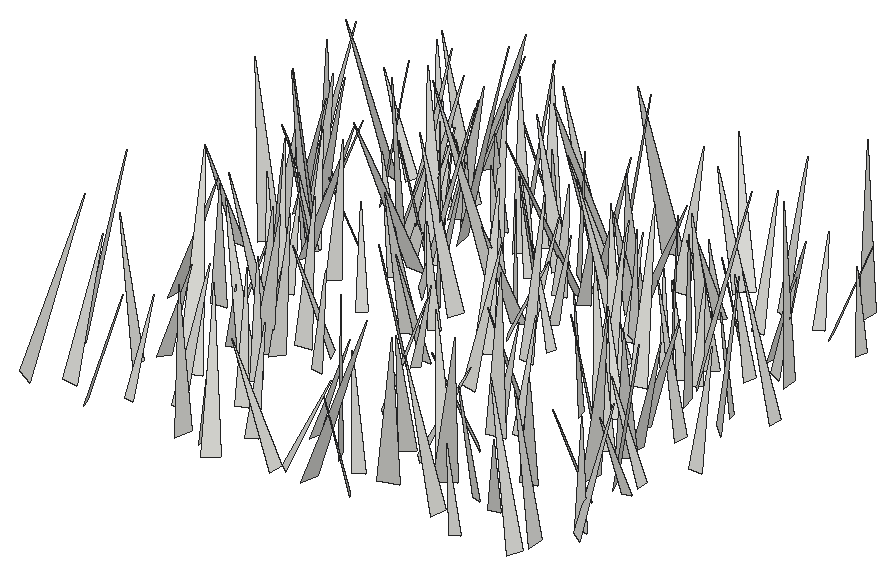
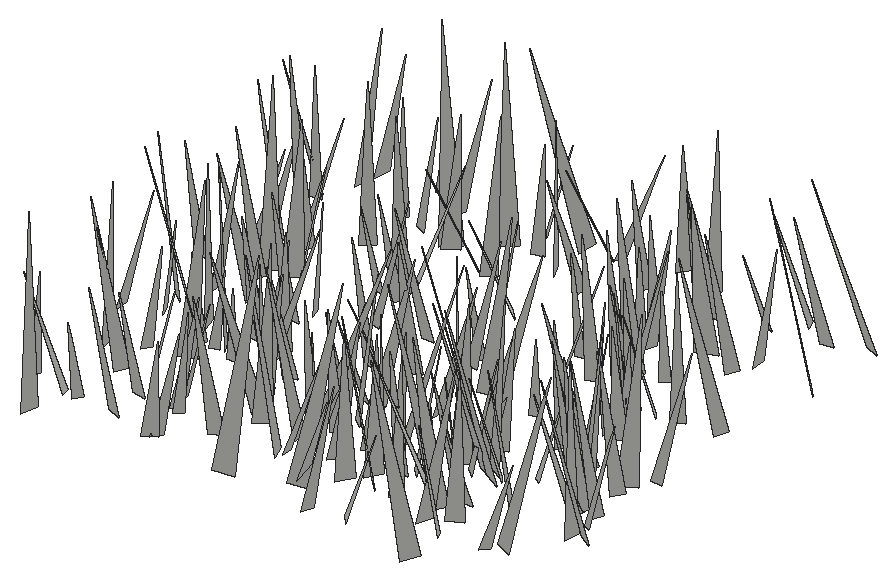
# SketchUp Ruby script. Lengths in inches.
U = 1.inch
M = Sketchup.active_model
def pt(a) = Geom::Point3d.new(a.map { |v| v * U })
def face(e, loops, mat)
  f = e.add_face(loops[0].map { |a| pt(a) })
  loops[1..].each { |l| e.add_face(l.map { |a| pt(a) }).erase! }
  f.material = f.back_material = mat if mat
  f
end
# faces: each face lists its corners as indices into pts; further lists are holes
def faces(e, pts, list, mat = nil) = list.each { |f| face(e, (f[0].is_a?(Array) ? f : [f]).map { |l| l.map { |i| pts[i] } }, mat) }
# xy, xz, yz: faces in a plane at the given z, y or x. An outline is a flat list of corners, or four numbers for a rectangle; further outlines are holes
def ring(l) = l.size == 4 ? [[l[0], l[1]], [l[2], l[1]], [l[2], l[3]], [l[0], l[3]]] : l.each_slice(2).to_a
def flat(e, list, mat, &to3) = list.each { |f| face(e, (f[0].is_a?(Array) ? f : [f]).map { |l| ring(l).map { |u, v| to3.(u, v) } }, mat) }
def xy(e, z, list, mat = nil) = flat(e, list, mat) { |x, y| [x, y, z] }
def xz(e, y, list, mat = nil) = flat(e, list, mat) { |x, z| [x, y, z] }
def yz(e, x, list, mat = nil) = flat(e, list, mat) { |y, z| [x, y, z] }
def lines(e, pts, list) = list.each { |a, b| e.add_line(pt(pts[a]), pt(pts[b])) }
# prism: a flat outline (further loops are holes) pulled along v
def prism(e, loops, v, mat = nil)
  f = face(e, loops, mat); d = Geom::Vector3d.new(v.map { |x| x * U })
  f.pushpull(f.normal.samedirection?(d) ? d.length : -d.length)
end
def box(e, o, s, mat = nil) = prism(e, [[o, [o[0] + s[0], o[1], o[2]], [o[0] + s[0], o[1] + s[1], o[2]], [o[0], o[1] + s[1], o[2]]]], [0, 0, s[2]], mat)
def at(x, y, z, deg = 0) = Geom::Transformation.translation(pt([x, y, z])) * Geom::Transformation.rotation(ORIGIN, Z_AXIS, deg.degrees)
def axes(o, x, y, z) = Geom::Transformation.new([*x, 0, *y, 0, *z, 0, *pt(o).to_a, 1])
def part(name) = M.definitions.add(name)
# library, detail: a bought-in or finely detailed component or shape, given as its bounding box
def library(name, o, s) = part(name).tap { |d| box(d.entities, o, s) }
def detail(e, o, s) = box(e.add_group.entities, o, s)
def put(e, d, t, mat = nil) = e.add_instance(d, t).tap { |i| i.material = mat if mat }
def group(e, t, mat = nil) = e.add_group.tap { |g| g.transformation = t; g.material = mat if mat }.entities
root = M.entities
c1 = part("fur_instance\#9")
p = [[0.8125,0,1.79],[0.67,-0.02,1.48],[0,-0.11,0],[0,0.11,0]]
faces(c1.entities,p,[[0,1,2,3]])
put(root,c1,axes([517.21,158.68,-21.66],[5.69628,-2.00129,2.37758],[-1.98509,-6.1627,-0.4314],[-2.39112,0.34864,6.02217]))
put(root,c1,axes([525.48,158.79,-21.66],[-5.10669,0.68056,0.36828],[0.71376,5.09217,0.48729],[0.29888,-0.53268,5.12875]))
put(root,c1,axes([509.02,157.88,-21.66],[4.30125,1.72732,0.68489],[1.69718,-4.35514,0.32517],[-0.75649,0.05042,4.6237]))
put(root,c1,axes([520.79,157.32,-21.66],[-4.49131,4.50007,0.95246],[4.50728,4.57122,-0.34355],[0.91773,-0.42777,6.34858]))
put(root,c1,axes([531.84,159.24,-21.66],[-3.00946,-2.45302,0.73779],[-2.54129,3.00205,-0.38468],[0.32167,0.76736,3.86344]))
put(root,c1,axes([518.95,158.54,-21.66],[-3.597,-0.64897,1.74683],[-0.97146,3.89365,-0.55385],[1.59023,0.91068,3.61287]))
put(root,c1,axes([541.32,159.27,-21.66],[1.53479,-3.08573,1.52348],[-3.30012,-1.79268,-0.30636],[-0.97569,1.2095,3.43271]))
put(root,c1,axes([528.25,159.17,-21.66],[7.76844,-0.71206,0.72464],[-0.74639,-7.79129,0.34557],[-0.68922,0.41169,7.79335]))
put(root,c1,axes([503.29,158.16,-21.66],[3.5873,6.66463,1.07182],[6.75002,-3.55215,-0.50434],[-0.05834,-1.18311,7.55193]))
put(root,c1,axes([525.89,159.3,-21.66],[2.47782,3.1575,0.0552],[3.13992,-2.45577,-0.47176],[0.33732,-0.3344,3.98583]))
put(root,c1,axes([532.87,162.28,-21.66],[3.4393,-6.56896,1.063],[-6.65437,-3.3911,0.57422],[0.02233,1.20797,7.39258]))
put(root,c1,axes([506.24,159.51,-21.66],[-0.03084,5.75903,1.17934],[5.85206,0.14189,-0.53988],[0.55736,-1.17118,5.73375]))
put(root,c1,axes([538.45,161.01,-21.66],[-6.00997,1.04438,1.22572],[1.13938,6.10462,0.38513],[1.13796,-0.59647,6.08787]))
put(root,c1,axes([546.26,159.875,-21.66],[-6.22467,1.67352,0.58559],[1.62437,6.23957,-0.56507],[0.71064,0.39649,6.42089]))
put(root,c1,axes([546.57,161.78,-21.66],[5.59524,-0.57904,3.08549],[-0.36766,-6.38318,-0.53118],[-3.11775,-0.28642,5.59999]))
put(root,c1,axes([511.12,160.11,-21.66],[1.03899,3.82207,0.22987],[3.79032,-1.06041,0.49963],[-0.54276,-0.08876,3.92914]))
put(root,c1,axes([521.38,161.21,-21.66],[2.89571,-2.97183,2.13904],[-3.49598,-3.05481,0.48854],[-1.08874,1.90494,4.12046]))
put(root,c1,axes([530.41,162.06,-21.66],[1.59272,-3.9303,2.28796],[-4.37909,-1.9795,-0.352],[-1.22702,1.96293,4.22612]))
put(root,c1,axes([541.33,163.7,-21.66],[1.84889,-3.8875,0.07331],[-3.87281,-1.83403,0.41727],[0.34554,0.24513,4.2845]))
put(root,c1,axes([514.63,161.35,-21.66],[0.44242,5.64748,1.29703],[5.78226,-0.34572,-0.46699],[0.37666,-1.32609,5.6455]))
put(root,c1,axes([536,164.81,-21.66],[5.23004,-6.31048,0.45418],[-6.32662,-5.22094,0.31214],[-0.04891,0.54893,8.19012]))
put(root,c1,axes([527.96,163.07,-21.66],[5.01686,3.02729,2.73746],[3.17963,-5.61852,0.38618],[-2.55892,-1.04628,5.84673]))
put(root,c1,axes([539.24,164.29,-21.66],[1.51862,3.68557,2.40948],[4.21899,-1.94756,0.31991],[-1.2606,-2.07817,3.97332]))
put(root,c1,axes([524.69,164.1875,-21.66],[4.46137,-0.22154,0.62784],[-0.29219,-4.4737,0.49769],[-0.59824,0.53291,4.43905]))
put(root,c1,axes([547.81,165.39,-21.66],[0.13174,-4.85064,1.64659],[-5.10405,0.01535,0.4536],[0.43432,1.65178,4.83118]))
put(root,c1,axes([531.17,166.6,-21.66],[3.50702,-4.68842,0.88051],[-4.69288,-3.58696,-0.4079],[-0.85643,0.45629,5.84073]))
put(root,c1,axes([508.36,164.66,-21.66],[-5.56537,0.35389,1.01892],[0.25962,5.63719,-0.53984],[1.04691,0.48332,5.55042]))
put(root,c1,axes([548.24,164.44,-21.66],[2.85218,4.71528,1.10181],[4.83661,-2.83604,-0.38317],[-0.23454,-1.14272,5.49745]))
put(root,c1,axes([517.9375,164.33,-21.66],[-0.91047,5.0165,1.03079],[5.11456,0.83694,0.44447],[-0.2628,-1.09133,5.07905]))
put(root,c1,axes([535.75,165.17,-21.66],[2.97491,-4.25566,3.74848],[-5.0806,-3.88069,-0.37363],[-2.51977,2.80026,5.17891]))
put(root,c1,axes([509.08,166.65,-21.66],[4.36325,-2.68491,0.18726],[-2.69098,-4.34538,0.39756],[0.04948,0.43666,5.1077]))
put(root,c1,axes([502.97,165.3,-21.66],[5.7382,5.20942,1.87337],[5.41352,-5.84467,-0.3291],[-1.15821,-1.50876,7.74318]))
put(root,c1,axes([540.72,168.36,-21.66],[2.46673,-5.38252,0.46134],[-5.39282,-2.42347,0.55987],[0.31917,0.65147,5.89431]))
put(root,c1,axes([532.47,166.27,-21.66],[3.00056,3.161,0.00616],[3.13284,-2.97269,-0.58633],[0.42105,-0.40809,4.31874]))
put(root,c1,axes([545.46,169.32,-21.66],[-2.21382,-3.77344,0.32599],[-3.76288,2.23425,0.30817],[0.43109,0.1241,4.36404]))
put(root,c1,axes([512.21,165.71,-21.66],[-3.14428,7.71271,0.49149],[7.72648,3.12546,0.38342],[-0.17032,-0.59964,8.32018]))
put(root,c1,axes([516.44,167.86,-21.66],[-4.17339,1.81444,1.20525],[1.74242,4.34394,-0.50613],[1.30721,0.0026,4.52253]))
put(root,c1,axes([534.71,170.26,-21.66],[-3.28468,-3.33783,0.1825],[-3.30088,3.27904,0.56182],[0.52783,-0.26523,4.64915]))
put(root,c1,axes([515.92,167.7,-21.66],[-6.2227,2.39174,0.32304],[2.36421,6.22042,-0.51348],[0.48507,0.36431,6.64671]))
put(root,c1,axes([512,170.68,-21.66],[1.97582,-3.11414,0.08334],[-3.10691,-1.9626,0.3224],[0.22782,0.24287,3.67393]))
put(root,c1,axes([547.16,171.4,-21.66],[0.58704,-3.79537,0.45103],[-3.78334,-0.64184,-0.47675],[-0.5428,0.36891,3.81079]))
put(root,c1,axes([514.3125,171.22,-21.66],[4.31409,-4.88001,1.43702],[-5.06352,-4.30068,0.59646],[-0.49016,1.47666,6.48614]))
put(root,c1,axes([543.75,171.66,-21.66],[6.97924,-1.80721,1.76653],[-1.77915,-7.19853,-0.33521],[-1.79479,0.10824,7.20163]))
put(root,c1,axes([526.32,169.87,-21.66],[3.1839,3.43631,0.24845],[3.39454,-3.18669,0.57383],[-0.5891,0.20968,4.64932]))
put(root,c1,axes([518.89,171.69,-21.66],[0.06663,3.86387,1.64805],[4.18879,0.06273,-0.31643],[0.31563,-1.6482,3.85147]))
put(root,c1,axes([545.68,171.99,-21.66],[5.68987,2.39384,1.65752],[2.61602,-5.80047,-0.60296],[-1.2784,-1.21517,6.14342]))
put(root,c1,axes([515.33,171.69,-21.66],[-4.36102,2.95909,2.58691],[3.11538,4.95832,-0.41976],[2.39639,-1.06094,5.25343]))
put(root,c1,axes([534.66,172.28,-21.66],[-1.49682,6.02983,3.22428],[6.74332,1.8484,-0.32627],[1.1325,-3.03643,6.20426]))
put(root,c1,axes([513.74,172.29,-21.66],[3.88682,0.49651,1.01606],[0.42112,-4.01087,0.34905],[-1.04955,0.22945,3.90283]))
put(root,c1,axes([547.17,173.17,-21.66],[-4.29082,0.07848,0.62907],[0.12494,4.3243,0.31276],[0.62151,-0.32753,4.28013]))
put(root,c1,axes([504.15,174.11,-21.66],[6.51578,-0.90085,0.09034],[-0.89347,-6.50413,-0.41604],[-0.1463,-0.39981,6.56459]))
put(root,c1,axes([518.3,174.24,-21.66],[-4.34148,-1.68145,0.56308],[-1.64517,4.37512,0.38015],[0.66161,-0.1544,4.64018]))
put(root,c1,axes([543.86,175.57,-21.66],[3.44417,-6.15496,0.43731],[-6.17002,-3.42915,0.33004],[0.07525,0.54268,7.04535]))
put(root,c1,axes([512.47,174.1875,-21.66],[-6.25427,-0.78477,1.30734],[-0.71032,6.38344,0.43371],[1.34924,-0.27711,6.28838]))
put(root,c1,axes([533.98,173.38,-21.66],[3.92282,-1.4058,1.44453],[-1.66907,-4.03753,0.60333],[-1.1301,1.0833,4.1232]))
put(root,c1,axes([507.6,174.75,-21.66],[1.5026,-5.2869,1.47769],[-5.48951,-1.44343,0.41772],[0.01326,1.53554,5.48039]))
put(root,c1,axes([515.98,173.75,-21.66],[-1.18817,5.57554,2.26119],[5.96275,1.39894,-0.31626],[0.80332,-2.13721,5.69196]))
put(root,c1,axes([535.79,173.29,-21.66],[0.78964,4.34465,0.57519],[4.335,-0.86018,0.54605],[-0.64386,-0.46311,4.38193]))
put(root,c1,axes([511.11,175.375,-21.66],[3.01124,-3.84874,1.35887],[-4.04465,-3.04041,0.35153],[-0.54781,1.29229,4.87409]))
put(root,c1,axes([523.21,176.34,-21.66],[-3.17607,-4.40082,1.193],[-4.40846,3.33508,0.56622],[1.16445,0.62283,5.3976]))
put(root,c1,axes([509.4,174.93,-21.66],[3.16954,2.48643,0.53995],[2.54162,-3.13416,-0.48689],[-0.1185,-0.71733,3.99891]))
put(root,c1,axes([540.9375,175.87,-21.66],[-4.28874,-2.62611,1.19653],[-2.76089,4.3576,-0.33198],[0.84,0.91449,5.01792]))
put(root,c1,axes([532.98,177.26,-21.66],[-1.82356,-4.42835,0.39133],[-4.41286,1.85435,0.42054],[0.53859,0.19978,4.77062]))
put(root,c1,axes([541.95,175.36,-21.66],[-4.3858,5.26104,2.02142],[5.54364,4.48874,0.34523],[1.01623,-1.78118,6.84066]))
put(root,c1,axes([543.71,176.92,-21.66],[5.53978,-0.90724,0.62547],[-0.85463,-5.56113,-0.49688],[-0.69563,-0.39269,5.59154]))
put(root,c1,axes([524.07,177.5,-21.66],[-0.19346,-4.85951,0.89963],[-4.92735,0.1202,-0.41034],[-0.38132,0.91231,4.84602]))
put(root,c1,axes([524.06,176.43,-21.66],[3.08181,-1.73974,0.98019],[-1.88437,-3.1302,0.36886],[-0.66077,0.81254,3.51969]))
put(root,c1,axes([528.84,176.48,-21.66],[0.94432,5.62245,1.27282],[5.76049,-0.87093,-0.42662],[0.22085,-1.32412,5.68522]))
put(root,c1,axes([548.88,177.07,-21.66],[-0.27729,4.76979,1.49646],[4.98187,0.38774,-0.31274],[0.41383,-1.47171,4.7676]))
put(root,c1,axes([510.15,177.32,-21.66],[3.4021,4.35261,1.87369],[4.47593,-3.70904,0.48912],[-1.55627,-1.15238,5.50275]))
put(root,c1,axes([520.65,179.97,-21.66],[2.01145,-6.31603,1.30369],[-6.40118,-2.12156,-0.40211],[-0.78536,1.11557,6.61638]))
put(root,c1,axes([510.41,177.15,-21.66],[-3.8761,2.85036,0.12124],[2.83481,3.87102,-0.37744],[0.32105,0.23257,4.79648]))
put(root,c1,axes([537.44,178.4,-21.66],[-4.30965,-1.39305,1.63599],[-1.58025,4.5392,-0.29767],[1.45598,0.80324,4.51941]))
put(root,c1,axes([542.13,179.65,-21.66],[5.3173,-1.56529,0.48292],[-1.59322,-5.32309,0.28875],[-0.38078,0.41424,5.53538]))
put(root,c1,axes([510.38,179.04,-21.66],[-2.95191,2.4359,0.97471],[2.3622,3.10602,-0.60836],[1.1418,-0.12828,3.77853]))
put(root,c1,axes([509.24,179.23,-21.66],[3.60121,-2.60608,3.3834],[-3.59297,-4.24118,0.55747],[-2.30861,2.53545,4.41017]))
put(root,c1,axes([545.16,180.07,-21.66],[-5.94659,0.26274,1.16381],[0.1992,6.05181,-0.34844],[1.17635,0.30341,5.94219]))
put(root,c1,axes([539.91,179.56,-21.66],[-2.40389,3.30252,0.08348],[3.28439,2.37806,0.4999],[-0.35549,-0.36124,4.05406]))
put(root,c1,axes([503.31,182.49,-21.66],[-0.2394,-4.99537,0.47277],[-5.01072,0.21306,-0.28607],[-0.26442,0.48521,4.99291]))
put(root,c1,axes([516.04,180.36,-21.66],[-1.47936,3.73163,0.54523],[3.76451,1.42617,0.45319],[-0.22551,-0.67216,3.98851]))
put(root,c1,axes([521.75,181.41,-21.66],[-1.38179,3.78074,1.32931],[4.00762,1.30133,0.46468],[-0.00636,-1.40818,3.99842]))
put(root,c1,axes([538.19,180.24,-21.66],[-0.0106,6.43156,0.96228],[6.47441,-0.07994,0.60561],[-0.61077,-0.95901,6.403]))
put(root,c1,axes([526.5625,180.99,-21.66],[-2.92394,5.35838,1.35906],[5.44647,3.05552,-0.32925],[0.94614,-1.02969,6.09534]))
put(root,c1,axes([546.47,182.7,-21.66],[-3.30417,-4.76212,3.2823],[-5.25525,4.05058,0.5865],[2.41528,2.29867,5.7664]))
put(root,c1,axes([508.65,184.03,-21.66],[-3.91635,-3.27614,1.36892],[-3.24396,4.13005,0.60351],[1.44353,0.39293,5.07017]))
put(root,c1,axes([511.65,182.64,-21.66],[4.3952,-2.19196,2.60814],[-2.70598,-4.83259,0.49862],[-2.06997,1.6632,4.88608]))
put(root,c1,axes([529.59,181.99,-21.66],[0.8824,6.11345,1.2337],[6.18895,-1.01221,0.58924],[-0.77016,-1.12963,6.14863]))
put(root,c1,axes([525.81,185.875,-21.66],[1.38462,-5.25865,0.1546],[-5.22749,-1.39323,-0.57157],[-0.5921,0.00308,5.40776]))
put(root,c1,axes([507.93,184.95,-21.66],[2.18541,-3.04998,0.78828],[-3.02604,-2.29919,-0.50659],[-0.87571,0.3334,3.71777]))
put(root,c1,axes([508.04,183.92,-21.66],[6.4862,-0.82849,0.61771],[-0.87391,-6.49276,0.46816],[-0.55158,0.54452,6.52212]))
put(root,c1,axes([504.5625,184.26,-21.66],[-4.39266,5.33205,2.64396],[5.82364,4.52851,0.54275],[1.2274,-2.40386,6.88706]))
put(root,c1,axes([526.33,183.93,-21.66],[3.11612,2.14822,0.04863],[2.13222,-3.08072,-0.53874],[0.26618,-0.47091,3.74631]))
put(root,c1,axes([515.29,187.39,-21.66],[-0.22294,-7.81188,0.28991],[-7.80547,0.20653,-0.4373],[-0.42917,0.30182,7.80282]))
put(root,c1,axes([542.3,184.4,-21.66],[5.88559,1.89129,2.87248],[1.95642,-6.52369,0.2867],[-2.82853,-0.57687,6.17535]))
put(root,c1,axes([530.08,184.23,-21.66],[-3.96056,0.86775,0.15545],[0.85071,3.94968,-0.37345],[0.23119,0.33194,4.03727]))
put(root,c1,axes([521.53,184.12,-21.66],[-6.69944,1.03913,0.45559],[1.00559,6.70154,-0.49804],[0.5255,0.42362,6.76123]))
put(root,c1,axes([545.92,184.85,-21.66],[-3.70453,-1.18645,1.17686],[-1.32576,3.8289,-0.31316],[1.01735,0.66938,3.87726]))
put(root,c1,axes([506.85,185.63,-21.66],[-6.68895,-1.28776,2.75903],[-1.15,7.23488,0.5888],[2.81923,-0.10417,6.78629]))
put(root,c1,axes([519.43,184.79,-21.66],[4.46233,4.90899,2.88894],[5.22756,-4.98695,0.39938],[-2.26203,-1.84084,6.62202]))
put(root,c1,axes([504.38,185.57,-21.66],[3.71133,-3.4553,1.19556],[-3.62183,-3.7076,0.52772],[-0.50083,1.20708,5.04327]))
put(root,c1,axes([514.78,185.7,-21.66],[2.55776,-3.86723,2.22173],[-4.13899,-3.01226,-0.47827],[-1.66143,1.55064,4.61182]))
put(root,c1,axes([535.6,184.43,-21.66],[-5.07407,3.61415,0.85454],[3.5922,5.14344,-0.42375],[0.94256,-0.14624,6.2152]))
put(root,c1,axes([539.35,186.17,-21.66],[5.6621,3.46946,2.68851],[3.90579,-5.98471,-0.5026],[-2.00251,-1.86297,6.62147]))
put(root,c1,axes([538.04,184.07,-21.66],[-1.0825,6.58238,0.66021],[6.6005,1.02978,0.55528],[-0.44383,-0.73975,6.64764]))
put(root,c1,axes([517.63,184.99,-21.66],[5.42391,5.6075,1.42758],[5.74422,-5.4537,-0.40246],[-0.69711,-1.3092,7.79108]))
put(root,c1,axes([510.11,187.46,-21.66],[-1.91573,-3.10975,0.18965],[-3.07242,1.92263,0.49017],[0.51647,-0.09744,3.61944]))
put(root,c1,axes([535.43,185.87,-21.66],[-7.05219,-0.0174,0.36445],[-0.04272,7.04446,-0.49029],[0.36236,0.49184,7.03515]))
put(root,c1,axes([548.85,186.08,-21.66],[-5.68888,-0.08485,0.69236],[-0.12916,5.71868,-0.36046],[0.68548,0.37338,5.67808]))
put(root,c1,axes([507.75,185.3,-21.66],[-3.18277,2.93848,0.48438],[2.88307,3.21784,-0.5768],[0.74643,0.10079,4.29324]))
put(root,c1,axes([505.79,187.72,-21.66],[-4.21383,-5.23135,2.06774],[-5.35043,4.52497,0.54449],[1.7365,1.24763,6.69529]))
put(root,c1,axes([539.85,186.875,-21.66],[-1.79664,3.17113,0.9039],[3.29721,1.71578,0.53432],[-0.03822,-1.04932,3.60534]))
put(root,c1,axes([541.16,186.78,-21.66],[-2.54986,2.80817,1.27437],[2.87177,2.76487,-0.34653],[1.12374,-0.69377,3.77724]))
put(root,c1,axes([524.45,187.15,-21.66],[2.05844,3.54151,1.67651],[3.74882,-2.33096,0.32115],[-1.13989,-1.27062,4.08367]))
put(root,c1,axes([526.73,186.17,-21.66],[1.45638,3.8911,0.37542],[3.87774,-1.48869,0.38679],[-0.49475,-0.21394,4.13668]))
put(root,c1,axes([527.83,187.33,-21.66],[3.18405,-1.52738,1.26596],[-1.78098,-3.25535,0.55182],[-0.87386,1.06936,3.48806]))
put(root,c1,axes([532.85,186.98,-21.66],[-1.4542,4.67664,1.33998],[4.76533,1.65076,-0.58976],[0.97884,-1.08869,4.86188]))
put(root,c1,axes([525.2,188.91,-21.66],[-3.25628,-4.53556,1.56998],[-4.60157,3.48952,0.53691],[1.36443,0.94415,5.55755]))
put(root,c1,axes([541.03,186.9,-21.66],[5.81873,5.70667,1.51485],[5.84557,-5.86726,-0.35074],[-0.83073,-1.31442,8.14252]))
put(root,c1,axes([540.54,188.99,-21.66],[3.54462,-5.56954,2.15269],[-5.7416,-3.86654,-0.54956],[-1.63946,1.49942,6.57891]))
put(root,c1,axes([537.79,187.46,-21.66],[-0.46969,3.55211,0.73396],[3.59032,0.35011,0.60316],[-0.51554,-0.79795,3.53189]))
put(root,c1,axes([513.28,188.33,-21.66],[2.89079,5.81329,3.19782],[6.3896,-3.37876,0.3661],[-1.787,-2.67707,6.48205]))
put(root,c1,axes([503.45,188.99,-21.66],[5.71322,-0.96407,0.62556],[-0.92485,-5.73993,-0.39936],[-0.68221,-0.29224,5.7802]))
put(root,c1,axes([533.83,188.78,-21.66],[0.99186,4.25892,2.03749],[4.71935,-0.95274,-0.30591],[-0.13232,-2.05608,4.36218]))
put(root,c1,axes([520.57,189.55,-21.66],[-7.92829,-1.68885,1.19775],[-1.65667,8.01779,0.33921],[1.24187,-0.08605,8.09907]))
put(root,c1,axes([514.54,189.48,-21.66],[-2.99975,-3.60869,1.08185],[-3.74003,3.01886,-0.30041],[0.45307,1.02732,4.68304]))
put(root,c1,axes([504.83,189.48,-21.66],[6.44965,-0.53992,1.19924],[-0.48241,-6.55498,-0.35669],[-1.22351,-0.26161,6.46237]))
put(root,c1,axes([504.86,189.12,-21.66],[5.24676,-2.59436,1.90695],[-2.83441,-5.4512,0.38233],[-1.5275,1.20389,5.84064]))
put(root,c1,axes([503.16,190.54,-21.66],[-1.78915,-3.44674,0.35763],[-3.41457,1.82215,0.479],[0.59044,0.09337,3.85378]))
put(root,c1,axes([526.71,191.61,-21.66],[-3.06964,-6.81398,0.3454],[-6.81954,3.05272,-0.38339],[-0.20825,0.47214,7.46364]))
put(root,c1,axes([512.125,188.9375,-21.66],[3.35941,2.47012,0.56366],[2.52325,-3.34641,-0.37364],[-0.22894,-0.63632,4.15301]))
put(root,c1,axes([543.62,189.75,-21.66],[-3.82053,1.38738,1.41647],[1.59253,3.97908,0.39802],[1.18113,-0.87734,4.0451]))
put(root,c1,axes([527.71,190.87,-21.66],[2.72527,-3.47225,0.02549],[-3.46346,-2.7159,0.33551],[0.24824,0.22715,4.40125]))
put(root,c1,axes([515.89,188.95,-21.66],[-4.29093,5.93832,1.73067],[6.14946,4.32229,0.41585],[0.66564,-1.65078,7.31456]))
put(root,c1,axes([504.95,189.91,-21.66],[4.62251,0.92588,0.22465],[0.9419,-4.60847,-0.38752],[-0.14333,-0.42437,4.69837]))
put(root,c1,axes([520.32,190.45,-21.66],[3.95695,-1.9726,1.7752],[-1.97238,-4.31833,-0.40205],[-1.77544,0.40099,4.40306]))
put(root,c1,axes([533.375,188.7,-21.66],[-0.09668,3.9627,0.07364],[3.92699,0.08582,0.53775],[-0.5359,-0.08606,3.92724]))
put(root,c1,axes([515.87,189.78,-21.66],[3.90442,0.1948,1.09665],[0.0575,-4.02752,0.51071],[-1.11233,0.47558,3.87577]))
put(root,c1,axes([513.73,188.83,-21.66],[3.6487,6.36792,1.23917],[6.47764,-3.65398,-0.29593],[-0.35515,-1.22351,7.3332]))
put(root,c1,axes([531.24,192.04,-21.66],[2.7716,-4.32676,0.73791],[-4.29866,-2.85215,-0.57784],[-0.88707,0.30254,5.10575]))
put(root,c1,axes([515.53,189.8,-21.66],[2.40724,3.27999,1.19788],[3.2967,-2.61439,0.53362],[-1.15108,-0.62824,4.03341]))
put(root,c1,axes([525.53,190.85,-21.66],[2.1664,-3.98299,1.68795],[-4.30586,-2.16689,0.41322],[-0.41582,1.68731,4.51516]))
put(root,c1,axes([517.49,192.04,-21.66],[-3.40896,-3.60182,1.17644],[-3.63778,3.55381,0.3393],[1.06005,0.61272,4.94762]))
put(root,c1,axes([512.63,189.44,-21.66],[3.66563,6.83822,1.35122],[6.90712,-3.76874,0.33492],[-0.93742,-1.02919,7.75151]))
put(root,c1,axes([546.21,191,-21.66],[-6.67663,-0.80436,2.4344],[-1.05353,7.05179,-0.55944],[2.33738,0.88086,6.7016]))
put(root,c1,axes([530.48,193.11,-21.66],[4.51111,-4.76568,1.07484],[-4.75985,-4.61702,-0.49408],[-1.1004,0.43419,6.54353]))
put(root,c1,axes([531.8,191.875,-21.66],[5.92157,-1.3609,0.111],[-1.36516,-5.91048,0.36315],[-0.02664,0.3788,6.06507]))
put(root,c1,axes([503.1,192.3,-21.66],[6.40054,-0.55178,2.21578],[-0.37829,-6.75939,-0.5905],[-2.25189,-0.43282,6.39709]))
put(root,c1,axes([544.67,191.29,-21.66],[2.00613,4.44684,1.43472],[4.67253,-1.91449,-0.59961],[-0.01581,-1.5549,4.84142]))
put(root,c1,axes([522.22,191.62,-21.66],[-1.64307,3.38565,0.94063],[3.51296,1.55882,0.52563],[-0.08077,-1.0745,3.72639]))
put(root,c1,axes([541,192.28,-21.66],[-2.98198,-2.20876,0.85448],[-2.34628,2.94214,-0.58291],[0.32208,0.98295,3.66484]))
put(root,c1,axes([543.05,193.3125,-21.66],[6.29896,-1.22347,0.37639],[-1.1888,-6.29213,-0.55798],[-0.47466,-0.47719,6.39237]))
put(root,c1,axes([527.08,193.13,-21.66],[6.44978,-0.00096,0.92482],[0.04605,-6.50733,-0.32793],[-0.92367,-0.33115,6.44144]))
put(root,c1,axes([536.98,193.7,-21.66],[-3.57828,-1.18752,0.86435],[-1.11493,3.67791,0.43741],[0.95617,-0.15551,3.74473]))
put(root,c1,axes([501.99,192.2,-21.66],[3.861,5.57007,1.34937],[5.71182,-3.87341,-0.35436],[-0.47072,-1.31331,6.76812]))
put(root,c1,axes([515.21,192.76,-21.66],[7.84011,2.17766,1.89393],[2.14429,-8.06482,0.39652],[-1.93163,-0.114,8.12726]))
put(root,c1,axes([507.1875,193.68,-21.66],[5.44742,2.57642,1.57153],[2.74581,-5.57692,-0.37485],[-1.25227,-1.0208,6.0143]))
put(root,c1,axes([518.24,192.72,-21.66],[-0.17119,5.69768,1.30234],[5.83131,0.07859,0.42267],[-0.39436,-1.31119,5.68456]))
put(root,c1,axes([523.24,193.85,-21.66],[-5.24229,2.67543,1.59997],[2.88849,5.34612,0.52444],[1.17239,-1.20849,5.86212]))
put(root,c1,axes([536.47,195.4,-21.66],[1.6071,-3.85332,0.26864],[-3.82652,-1.62792,-0.45895],[-0.52725,0.06941,4.14972]))
put(root,c1,axes([511.7,193.28,-21.66],[0.71871,3.7725,0.80138],[3.83913,-0.62217,-0.51422],[0.36739,-0.87844,3.80576]))
put(root,c1,axes([525.01,193.66,-21.66],[2.79154,3.79561,1.789],[3.98615,-3.06992,0.29332],[-1.31064,-1.25251,4.70248]))
put(root,c1,axes([513.9375,194.79,-21.66],[0.22689,-3.51122,0.97081],[-3.62685,-0.12635,0.39066],[0.3422,0.98893,3.49679]))
put(root,c1,axes([516.375,195.57,-21.66],[1.54796,-4.76639,0.70367],[-4.81569,-1.50748,0.38266],[0.1508,0.78667,4.99682]))
put(root,c1,axes([513.02,194.97,-21.66],[5.25974,-3.61511,1.15521],[-3.73911,-5.27428,0.51907],[-0.65007,1.0869,6.36116]))
put(root,c1,axes([526.51,195.35,-21.66],[-4.93591,-0.64757,0.62999],[-0.58328,4.95621,0.52453],[0.68994,-0.44273,4.95049]))
put(root,c1,axes([536.02,195.64,-21.66],[2.32734,-2.83374,0.7234],[-2.82694,-2.41664,-0.37171],[-0.74954,0.31569,3.64807]))
put(root,c1,axes([521.48,195.49,-21.66],[-0.96334,-4.21277,1.52504],[-4.43315,1.12201,0.29911],[0.64835,1.41239,4.31115]))
put(root,c1,axes([519.56,194.13,-21.66],[-5.3119,3.70536,1.5571],[3.75007,5.49761,-0.28937],[1.44609,-0.64586,6.4701]))
put(root,c1,axes([505.83,196.67,-21.66],[-2.53564,-6.45433,1.27855],[-6.57975,2.48748,-0.49186],[0.00081,1.3699,6.91708]))
put(root,c1,axes([522.91,198.66,-21.66],[1.39715,-7.46285,0.32526],[-7.45597,-1.41344,-0.40331],[-0.45656,0.24497,7.58179]))
put(root,c1,axes([526.97,195.8,-21.66],[6.97385,3.06548,2.09729],[3.25235,-7.19468,-0.2986],[-1.79388,-1.12684,7.61201]))
put(root,c1,axes([510.95,195.71,-21.66],[-2.98056,5.41129,1.99239],[5.72855,3.03527,0.32601],[0.65987,-1.90801,6.16924]))
put(root,c1,axes([518.79,195.14,-21.66],[4.76999,5.26227,1.90717],[5.37132,-5.00824,0.38463],[-1.57405,-1.14351,7.09199]))
put(root,c1,axes([513.47,194.72,-21.66],[5.3948,4.35682,0.5893],[4.31887,-5.42625,0.57994],[-0.82254,0.08385,6.9101]))
put(root,c1,axes([520.79,195.82,-21.66],[-5.28353,4.19242,1.51467],[4.2139,5.46353,-0.42331],[1.45386,-0.59977,6.73148]))
put(root,c1,axes([539.83,195.4375,-21.66],[0.07202,5.27236,0.64208],[5.29211,-0.12578,0.43929],[-0.45123,-0.63374,5.25452]))
put(root,c1,axes([512.72,196.95,-21.66],[-6.49588,1.72746,1.45223],[1.82521,6.62397,0.28488],[1.32729,-0.65455,6.71561]))
put(root,c1,axes([547.47,197.54,-21.66],[3.35457,-1.66316,1.27005],[-1.64462,-3.57909,-0.343],[-1.29397,0.23728,3.72849]))
put(root,c1,axes([531.97,196.49,-21.66],[-1.06035,5.5551,1.84187],[5.77115,1.30347,-0.60889],[0.97234,-1.67863,5.62252]))
put(root,c1,axes([506.85,197.47,-21.66],[-3.73085,2.02538,0.45172],[2.07172,3.68874,0.57157],[0.11914,-0.71871,4.20651]))
put(root,c1,axes([510.625,197.9375,-21.66],[3.65523,2.01923,0.98653],[2.16689,-3.66612,-0.52479],[-0.59594,-0.94526,4.14277]))
put(root,c1,axes([522.96,198.12,-21.66],[-3.66432,1.46778,0.50332],[1.5223,3.65057,0.437],[0.30055,-0.59495,3.9231]))
put(root,c1,axes([544.1875,198.31,-21.66],[4.46845,1.48023,0.19389],[1.49287,-4.43008,-0.58427],[0.00126,-0.6156,4.67084]))
put(root,c1,axes([528.1,200.52,-21.66],[1.76512,-7.95634,1.31885],[-8.03843,-1.84494,-0.37166],[-0.65291,1.20466,8.14131]))
put(root,c1,axes([542.9375,198.45,-21.66],[-2.61192,2.51011,0.78878],[2.46687,2.72278,-0.49597],[0.91509,-0.17543,3.58843]))
put(root,c1,axes([535.18,199.2,-21.66],[-4.286,2.05614,0.85108],[2.13965,4.31523,0.34994],[0.6115,-0.68765,4.74078]))
put(root,c1,axes([517.2,200.35,-21.66],[-2.83398,-2.56318,0.53676],[-2.6174,2.79801,-0.45803],[0.08496,0.70049,3.79362]))
put(root,c1,axes([539.5625,198.59,-21.66],[1.82838,5.64567,1.15342],[5.69001,-1.95997,0.57384],[-0.90985,-0.91206,5.90655]))
put(root,c1,axes([520.18,200.89,-21.66],[-5.09295,0.86723,1.4086],[1.03106,5.23004,0.50795],[1.29351,-0.75432,5.14123]))
put(root,c1,axes([510.1,201.84,-21.66],[6.42408,-3.63909,0.41323],[-3.66082,-6.40525,0.50369],[-0.11006,0.64215,7.36601]))
put(root,c1,axes([535.46,199.59,-21.66],[-3.60755,4.52257,0.00535],[4.517,3.60276,0.29145],[-0.22451,-0.18592,5.77782]))
put(root,c1,axes([544.48,202.01,-21.66],[7.21029,-1.27081,2.71678],[-1.16788,-7.70491,-0.50453],[-2.76259,-0.05954,7.30402]))
